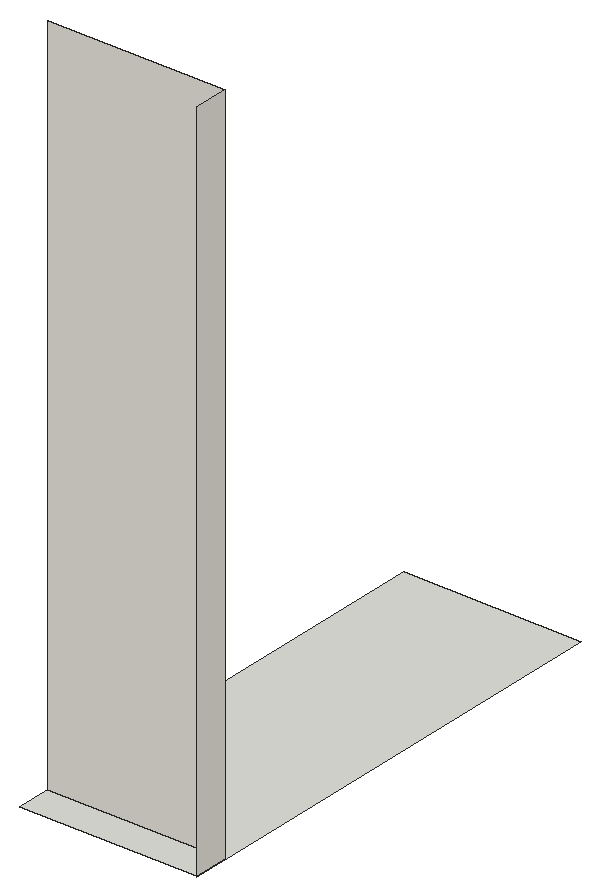
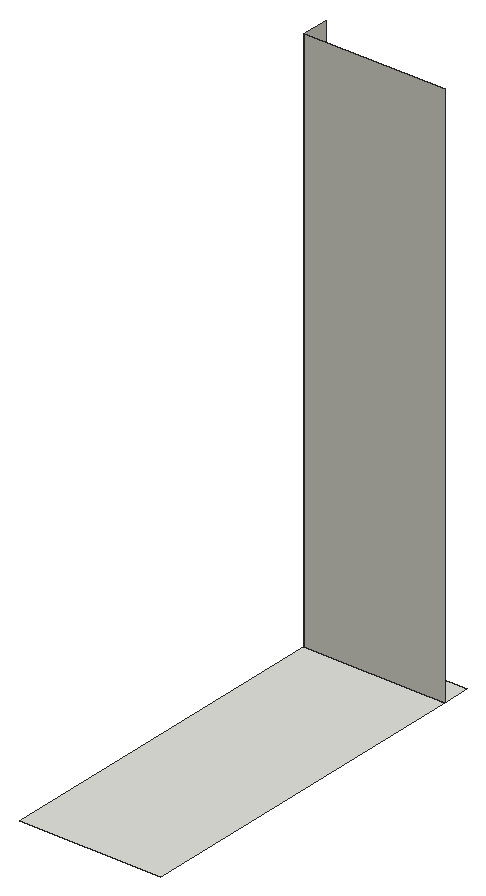
# SketchUp Ruby script. Lengths in inches.
U = 1.inch
M = Sketchup.active_model
def pt(a) = Geom::Point3d.new(a.map { |v| v * U })
def face(e, loops, mat)
  f = e.add_face(loops[0].map { |a| pt(a) })
  loops[1..].each { |l| e.add_face(l.map { |a| pt(a) }).erase! }
  f.material = f.back_material = mat if mat
  f
end
# faces: each face lists its corners as indices into pts; further lists are holes
def faces(e, pts, list, mat = nil) = list.each { |f| face(e, (f[0].is_a?(Array) ? f : [f]).map { |l| l.map { |i| pts[i] } }, mat) }
# xy, xz, yz: faces in a plane at the given z, y or x. An outline is a flat list of corners, or four numbers for a rectangle; further outlines are holes
def ring(l) = l.size == 4 ? [[l[0], l[1]], [l[2], l[1]], [l[2], l[3]], [l[0], l[3]]] : l.each_slice(2).to_a
def flat(e, list, mat, &to3) = list.each { |f| face(e, (f[0].is_a?(Array) ? f : [f]).map { |l| ring(l).map { |u, v| to3.(u, v) } }, mat) }
def xy(e, z, list, mat = nil) = flat(e, list, mat) { |x, y| [x, y, z] }
def xz(e, y, list, mat = nil) = flat(e, list, mat) { |x, z| [x, y, z] }
def yz(e, x, list, mat = nil) = flat(e, list, mat) { |y, z| [x, y, z] }
def lines(e, pts, list) = list.each { |a, b| e.add_line(pt(pts[a]), pt(pts[b])) }
# prism: a flat outline (further loops are holes) pulled along v
def prism(e, loops, v, mat = nil)
  f = face(e, loops, mat); d = Geom::Vector3d.new(v.map { |x| x * U })
  f.pushpull(f.normal.samedirection?(d) ? d.length : -d.length)
end
def box(e, o, s, mat = nil) = prism(e, [[o, [o[0] + s[0], o[1], o[2]], [o[0] + s[0], o[1] + s[1], o[2]], [o[0], o[1] + s[1], o[2]]]], [0, 0, s[2]], mat)
def at(x, y, z, deg = 0) = Geom::Transformation.translation(pt([x, y, z])) * Geom::Transformation.rotation(ORIGIN, Z_AXIS, deg.degrees)
def axes(o, x, y, z) = Geom::Transformation.new([*x, 0, *y, 0, *z, 0, *pt(o).to_a, 1])
def part(name) = M.definitions.add(name)
# library, detail: a bought-in or finely detailed component or shape, given as its bounding box
def library(name, o, s) = part(name).tap { |d| box(d.entities, o, s) }
def detail(e, o, s) = box(e.add_group.entities, o, s)
def put(e, d, t, mat = nil) = e.add_instance(d, t).tap { |i| i.material = mat if mat }
def group(e, t, mat = nil) = e.add_group.tap { |g| g.transformation = t; g.material = mat if mat }.entities
root = M.entities
M.materials.add("[Tile Limestone Large]").color = [237, 234, 224]
xy(root,17.625,[[76.4,137.79,111.84,144.7],[111.84,137.79,111.93,144.7],[76.4,144.7,111.93,233.86]])
xz(root,144.7,[[76.4,17.625,111.84,155.84]],"[Tile Limestone Large]")
yz(root,111.84,[[137.79,17.625,144.7,155.84]],"[Tile Limestone Large]")
